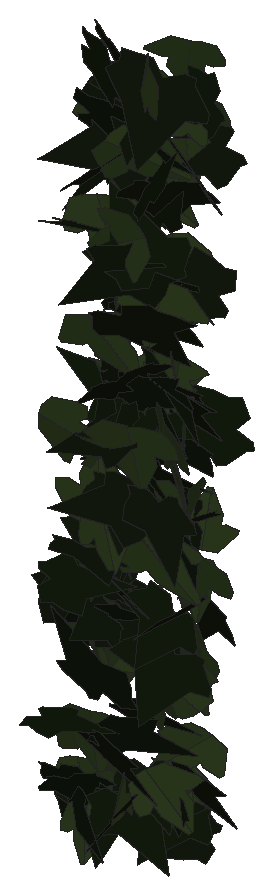
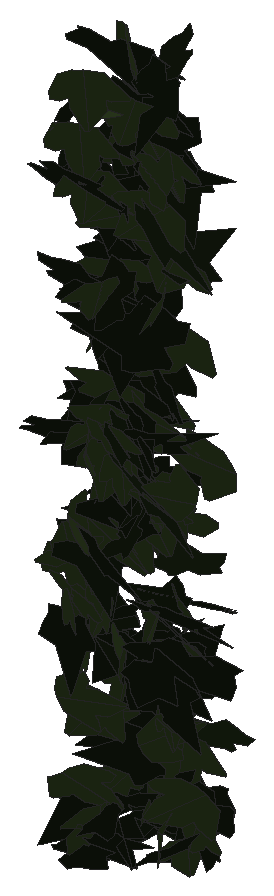
# SketchUp Ruby script. Lengths in inches.
U = 1.inch
M = Sketchup.active_model
def pt(a) = Geom::Point3d.new(a.map { |v| v * U })
def face(e, loops, mat)
  f = e.add_face(loops[0].map { |a| pt(a) })
  loops[1..].each { |l| e.add_face(l.map { |a| pt(a) }).erase! }
  f.material = f.back_material = mat if mat
  f
end
# faces: each face lists its corners as indices into pts; further lists are holes
def faces(e, pts, list, mat = nil) = list.each { |f| face(e, (f[0].is_a?(Array) ? f : [f]).map { |l| l.map { |i| pts[i] } }, mat) }
# xy, xz, yz: faces in a plane at the given z, y or x. An outline is a flat list of corners, or four numbers for a rectangle; further outlines are holes
def ring(l) = l.size == 4 ? [[l[0], l[1]], [l[2], l[1]], [l[2], l[3]], [l[0], l[3]]] : l.each_slice(2).to_a
def flat(e, list, mat, &to3) = list.each { |f| face(e, (f[0].is_a?(Array) ? f : [f]).map { |l| ring(l).map { |u, v| to3.(u, v) } }, mat) }
def xy(e, z, list, mat = nil) = flat(e, list, mat) { |x, y| [x, y, z] }
def xz(e, y, list, mat = nil) = flat(e, list, mat) { |x, z| [x, y, z] }
def yz(e, x, list, mat = nil) = flat(e, list, mat) { |y, z| [x, y, z] }
def lines(e, pts, list) = list.each { |a, b| e.add_line(pt(pts[a]), pt(pts[b])) }
# prism: a flat outline (further loops are holes) pulled along v
def prism(e, loops, v, mat = nil)
  f = face(e, loops, mat); d = Geom::Vector3d.new(v.map { |x| x * U })
  f.pushpull(f.normal.samedirection?(d) ? d.length : -d.length)
end
def box(e, o, s, mat = nil) = prism(e, [[o, [o[0] + s[0], o[1], o[2]], [o[0] + s[0], o[1] + s[1], o[2]], [o[0], o[1] + s[1], o[2]]]], [0, 0, s[2]], mat)
def at(x, y, z, deg = 0) = Geom::Transformation.translation(pt([x, y, z])) * Geom::Transformation.rotation(ORIGIN, Z_AXIS, deg.degrees)
def axes(o, x, y, z) = Geom::Transformation.new([*x, 0, *y, 0, *z, 0, *pt(o).to_a, 1])
def part(name) = M.definitions.add(name)
# library, detail: a bought-in or finely detailed component or shape, given as its bounding box
def library(name, o, s) = part(name).tap { |d| box(d.entities, o, s) }
def detail(e, o, s) = box(e.add_group.entities, o, s)
def put(e, d, t, mat = nil) = e.add_instance(d, t).tap { |i| i.material = mat if mat }
def group(e, t, mat = nil) = e.add_group.tap { |g| g.transformation = t; g.material = mat if mat }.entities
root = M.entities
M.materials.add("1026 AP 7946 SUNNY SIDE UP").color = [254, 231, 186]
M.materials.add("efeu1").color = [18, 25, 13]
M.materials.add("efeu2").color = [43, 57, 29]
c1 = part("ivyleaf_10")
p = [[0,0.5,-0.03],[-0.0625,2.02,-0.43],[-0.19,2.01,-0.46],[-0.54,1.05,-0.29],[-0.52,0.625,-0.18],[-0.83,0.76,-0.28],
  [-1.16,0.64,-0.33],[-1.15,0.33,-0.24],[-0.77,-0.39,0.02],[-0.3,-0.51,0.16],[0.04,-0.48,0.23],[-0.02,2.01,-0.4375],
  [-0.06,2.01,-0.43],[0.04,-0.49,0.23],[0.67,-0.49,0.14],[1.38,0.36,-0.2],[1.375,0.51,-0.24],[0.81,0.65,-0.19],
  [0.62,0.59,-0.15],[0.6,1.09,-0.28],[0.5,1.23,-0.31]]
faces(c1.entities,p,[[0,1,2,3,4,5,6,7,8,9,10],[11,12,0,13,14,15,16,17,18,19,20]],"efeu2")
c2 = part("ivyleaf_9")
p = [[1.54,2.16,1.25],[1.36,2.04,1.19],[-0.21,0.99,0.68],[-0.71,1.11,0.82],[-0.85,0.86,0.67],[-0.8,0.17,0.21],
  [-0.9,-0.01,0.1],[-0.67,-0.16,-0.02],[-0.08,-0.08,-0.05],[-0.03,-0.6,-0.4],[0.65,-0.88,-0.66],[0.83,-0.6,-0.49],
  [1.29,-0.42,-0.43],[1.8125,-0.07,-0.26],[1.21,0.44,0.15]]
faces(c2.entities,p,[[0,1,2,3,4,5,6,7,8,9,10,11,12,13,14]],"efeu1")
put(root,c1,axes([141.98,211.67,268.41],[0.3411,-0.04466,0.11048],[0.16001,-0.03763,-0.22788],[0.08887,0.23916,-0.01374]),"1026 AP 7946 SUNNY SIDE UP")
put(root,c2,axes([142.37,212.03,271.69],[-0.51179,-0.04689,0.03116],[-0.02985,-0.07688,-0.33075],[0.08274,-0.31774,0.07342]),"1026 AP 7946 SUNNY SIDE UP")
put(root,c2,axes([142.38,212.01,270.58],[0.16585,0.07044,-0.27143],[-0.35182,-0.13992,-0.13143],[-0.24626,0.24734,0.00497]),"1026 AP 7946 SUNNY SIDE UP")
put(root,c2,axes([142.32,212.13,270.93],[-0.05032,0.15512,-0.27609],[0.02205,-0.26931,-0.16335],[-0.4876,-0.02818,0.02111]),"1026 AP 7946 SUNNY SIDE UP")
put(root,c1,axes([141.97,211.8,268.92],[-0.39891,0.00207,-0.21595],[0.3263,-0.0443,-0.25942],[-0.04686,-0.3261,0.03193]),"1026 AP 7946 SUNNY SIDE UP")
put(root,c2,axes([142.06,211.26,268.57],[0.37583,0.06079,-0.02788],[-0.03131,-0.03229,-0.25282],[-0.10006,0.2384,-0.02562]),"1026 AP 7946 SUNNY SIDE UP")
put(root,c1,axes([142.29,211.69,270.94],[-0.40485,-0.03673,0.02647],[-0.03461,-0.02825,-0.26688],[0.06162,-0.25723,0.02398]),"1026 AP 7946 SUNNY SIDE UP")
put(root,c2,axes([142.41,211.94,271.52],[-0.39007,0.07794,-0.04071],[0.04506,-0.0412,-0.26629],[-0.13014,-0.24787,0.02982]),"1026 AP 7946 SUNNY SIDE UP")
put(root,c2,axes([142.42,212.125,277.55],[-0.42812,0.2333,-0.19837],[0.19927,-0.14921,-0.36919],[-0.43335,-0.29909,0.0262]),"1026 AP 7946 SUNNY SIDE UP")
put(root,c2,axes([141.96,211.89,271.05],[-0.1553,-0.19578,-0.34367],[0.27144,0.28452,-0.22376],[0.5426,-0.19837,0.01357]),"1026 AP 7946 SUNNY SIDE UP")
put(root,c1,axes([142.34,212.11,269.78],[0.03474,0.09893,0.29942],[-0.08598,-0.2849,0.10271],[0.47419,-0.0589,-0.00331]),"1026 AP 7946 SUNNY SIDE UP")
put(root,c1,axes([142.28,211.88,270.18],[-0.05171,-0.25295,-0.0237],[0.01452,0.02055,-0.26258],[0.39892,-0.03354,0.00649]),"1026 AP 7946 SUNNY SIDE UP")
put(root,c1,axes([142.18,211.77,273.24],[-0.02523,-0.13468,0.29495],[0.07676,0.28296,0.14122],[-0.49266,0.05099,0.0069]),"1026 AP 7946 SUNNY SIDE UP")
put(root,c1,axes([141.92,211.34,273.64],[-0.07651,0.00007,-0.36728],[0.49858,-0.1645,-0.04558],[-0.25629,-0.32002,0.02098]),"1026 AP 7946 SUNNY SIDE UP")
put(root,c2,axes([141.99,211.02,269.45],[0.23151,-0.20375,0.03077],[0.30705,0.12572,-0.1034],[0.10365,0.08268,0.23759]),"1026 AP 7946 SUNNY SIDE UP")
put(root,c2,axes([142.03,211.14,271.4375],[0.3609,-0.09301,-0.09777],[0.13489,0.24816,-0.03558],[0.1588,0.00058,0.25243]),"1026 AP 7946 SUNNY SIDE UP")
put(root,c2,axes([142.54,211.94,273.32],[-0.23259,0.23044,-0.01208],[-0.00128,-0.016,-0.28203],[-0.36292,-0.14763,0.00874]),"1026 AP 7946 SUNNY SIDE UP")
put(root,c2,axes([142.34,211.07,268.62],[0.23158,0.2003,-0.03003],[-0.01105,-0.03236,-0.25594],[-0.31833,0.14683,-0.01296]),"1026 AP 7946 SUNNY SIDE UP")
put(root,c1,axes([142.28,211.64,271.64],[0.29083,-0.15606,0.10948],[0.13347,-0.06553,-0.24965],[0.26606,0.20346,0.00557]),"1026 AP 7946 SUNNY SIDE UP")
put(root,c1,axes([142.48,211.77,270.63],[-0.40923,-0.15968,0.0214],[-0.00811,-0.03291,-0.31367],[0.25326,-0.25908,0.02454]),"1026 AP 7946 SUNNY SIDE UP")
put(root,c2,axes([142.11,211.33,268.22],[-0.00991,-0.02689,-0.31801],[0.48409,-0.03418,-0.00361],[-0.05307,-0.30671,0.02646]),"1026 AP 7946 SUNNY SIDE UP")
put(root,c1,axes([142.35,211.42,267.98],[0.20432,0.27023,-0.07488],[-0.02966,-0.07319,-0.30898],[-0.43965,0.13052,-0.01395]),"1026 AP 7946 SUNNY SIDE UP")
put(root,c2,axes([142.55,211.55,276.59],[-0.45066,-0.04883,0.00443],[0.07538,-0.28465,-0.03772],[0.01629,-0.03374,0.29714]),"1026 AP 7946 SUNNY SIDE UP")
put(root,c1,axes([142.36,211.65,270.33],[-0.09142,0.24804,-0.03639],[0.00938,-0.03632,-0.26266],[-0.39417,-0.05839,0.00219]),"1026 AP 7946 SUNNY SIDE UP")
put(root,c2,axes([142.32,211.8,268.09],[-0.12544,-0.31489,0.04124],[-0.00584,-0.0422,-0.33483],[0.49945,-0.07958,0.00644]),"1026 AP 7946 SUNNY SIDE UP")
put(root,c1,axes([142.46,211.41,269.37],[-0.52293,-0.04642,-0.00997],[0.02694,-0.05566,-0.34115],[0.06943,-0.32801,0.05729]),"1026 AP 7946 SUNNY SIDE UP")
put(root,c1,axes([142.5,211.71,268.19],[-0.02876,0.15992,-0.25655],[-0.04368,0.24839,0.16727],[0.46451,0.03326,-0.00015]),"1026 AP 7946 SUNNY SIDE UP")
put(root,c1,axes([142.35,211.9375,270.78],[0.35241,0.13023,-0.00815],[0.00541,-0.02308,-0.26624],[-0.20516,0.2231,-0.02102]),"1026 AP 7946 SUNNY SIDE UP")
put(root,c1,axes([142.14,212.2,278.06],[-0.10439,-0.02513,0.32624],[0.45519,-0.13836,0.05037],[0.20625,0.29264,0.05394]),"1026 AP 7946 SUNNY SIDE UP")
put(root,c2,axes([142.39,211.5,270.93],[0.30046,0.17784,-0.00707],[0.00972,-0.01818,-0.26842],[-0.27974,0.19038,-0.01693]),"1026 AP 7946 SUNNY SIDE UP")
put(root,c1,axes([142.51,211.76,273.21],[0.01338,-0.31658,0.13614],[0.00947,-0.13383,-0.32703],[0.54043,0.01018,0.00236]),"1026 AP 7946 SUNNY SIDE UP")
put(root,c2,axes([142.79,211.91,273.95],[-0.333,-0.21274,-0.0949],[-0.1267,-0.04771,0.3081],[-0.341,0.22547,-0.02179]),"1026 AP 7946 SUNNY SIDE UP")
put(root,c1,axes([142.45,212,271.54],[-0.2126,0.22431,-0.02991],[0.00855,-0.03207,-0.26973],[-0.35581,-0.1348,0.01138]),"1026 AP 7946 SUNNY SIDE UP")
put(root,c1,axes([142.28,211.74,276.72],[0.5058,0.00687,0.14965],[0.22859,-0.01239,-0.33121],[-0.00182,0.35271,-0.01248]),"1026 AP 7946 SUNNY SIDE UP")
put(root,c1,axes([142.34,212.05,277.56],[-0.43096,0.00456,-0.18907],[0.28373,-0.05432,-0.27927],[-0.05342,-0.32536,0.04202]),"1026 AP 7946 SUNNY SIDE UP")
put(root,c2,axes([142.35,211.76,274.55],[-0.04657,0.15349,0.28758],[0.09403,-0.2718,0.15941],[0.49079,0.06664,-0.00325]),"1026 AP 7946 SUNNY SIDE UP")
put(root,c2,axes([142.5,211.71,279.25],[0.42137,-0.10113,-0.20957],[-0.31287,0.0455,-0.29389],[0.17071,0.33301,-0.02133]),"1026 AP 7946 SUNNY SIDE UP")
put(root,c1,axes([142.48,211.83,276.11],[-0.05506,0.28152,-0.16174],[0.02936,-0.1575,-0.29318],[-0.50723,-0.03968,0.00059]),"1026 AP 7946 SUNNY SIDE UP")
put(root,c2,axes([142.77,211.8,277.84],[-0.0214,-0.15522,-0.31691],[-0.07455,-0.3032,0.15845],[-0.53539,0.04842,-0.0094]),"1026 AP 7946 SUNNY SIDE UP")
put(root,c1,axes([142.54,211.74,278.22],[0.52281,-0.1236,-0.00956],[-0.02872,-0.02459,-0.36432],[0.19269,0.33169,-0.02835]),"1026 AP 7946 SUNNY SIDE UP")
put(root,c2,axes([142.58,211.53,270.92],[-0.15347,-0.1387,0.20366],[-0.09559,-0.1931,-0.17095],[0.36854,-0.10784,0.04047]),"1026 AP 7946 SUNNY SIDE UP")
put(root,c2,axes([142.78,211.1875,277.79],[-0.02929,0.36162,0.00368],[-0.01242,0.00111,-0.37294],[-0.56849,-0.01866,0.00796]),"1026 AP 7946 SUNNY SIDE UP")
put(root,c1,axes([142.94,211.71,274.18],[0.15447,0.03666,0.32107],[-0.48995,0.04831,0.09568],[-0.05576,-0.32299,0.0488]),"1026 AP 7946 SUNNY SIDE UP")
put(root,c2,axes([142.83,212.26,273.84],[-0.39672,0.13381,-0.09281],[0.10282,-0.06959,-0.29306],[-0.2326,-0.25898,0.02876]),"1026 AP 7946 SUNNY SIDE UP")
put(root,c1,axes([142.77,211.67,272.76],[-0.31169,-0.15376,0.10483],[-0.07505,-0.10281,-0.25425],[0.28083,-0.19813,0.0484]),"1026 AP 7946 SUNNY SIDE UP")
put(root,c2,axes([142.87,211.0625,270.16],[0.24883,-0.14306,0.30101],[-0.30423,0.22095,0.22008],[-0.41268,-0.24914,0.01925]),"1026 AP 7946 SUNNY SIDE UP")
put(root,c2,axes([142.45,211.3,271.96],[-0.10405,-0.24607,0.08055],[0.29188,-0.10239,-0.16774],[0.28316,0.01512,0.20251]),"1026 AP 7946 SUNNY SIDE UP")
put(root,c1,axes([142.68,211.29,272.61],[0.58544,0.09555,0.0268],[-0.05453,0.03324,0.39396],[0.14562,-0.37171,0.03979]),"1026 AP 7946 SUNNY SIDE UP")
put(root,c2,axes([142.85,212.28,274.3],[-0.25362,0.16214,-0.16063],[0.15152,-0.12481,-0.23574],[-0.32072,-0.18719,0.01565]),"1026 AP 7946 SUNNY SIDE UP")
put(root,c1,axes([142.6,211.33,275.3],[-0.48086,-0.09389,-0.16806],[0.26727,-0.0064,-0.32556],[0.12544,-0.3463,0.04941]),"1026 AP 7946 SUNNY SIDE UP")
put(root,c2,axes([142.47,211.625,271.43],[0.1434,-0.16128,0.19188],[0.18335,-0.1478,-0.1906],[0.34251,0.14664,0.0217]),"1026 AP 7946 SUNNY SIDE UP")
put(root,c2,axes([143.125,211.2,273.98],[-0.44703,0.18032,0.0289],[-0.06504,-0.01503,-0.34506],[-0.27922,-0.28518,0.03412]),"1026 AP 7946 SUNNY SIDE UP")
put(root,c2,axes([142.62,212.15,272.87],[0.32789,-0.20444,-0.06832],[-0.09814,0.02914,-0.29979],[0.3228,0.21652,-0.02175]),"1026 AP 7946 SUNNY SIDE UP")
put(root,c1,axes([142.85,212.12,273.74],[-0.18542,-0.24817,-0.01169],[0.03632,0,-0.28224],[0.38884,-0.11834,0.02079]),"1026 AP 7946 SUNNY SIDE UP")
put(root,c2,axes([142.65,211.17,279.41],[0.42453,-0.20228,-0.20018],[-0.21595,0.13801,-0.34583],[0.38313,0.30193,0.02689]),"1026 AP 7946 SUNNY SIDE UP")
put(root,c2,axes([142.4375,211.87,275.48],[0.18233,0.0042,0.32775],[0.49802,0.03045,-0.11917],[-0.04724,0.33722,0.00866]),"1026 AP 7946 SUNNY SIDE UP")
put(root,c2,axes([142.55,211.94,269.41],[0.32148,-0.03205,0.15256],[0.23518,0.00104,-0.21223],[0.03984,0.25255,0.02173]),"1026 AP 7946 SUNNY SIDE UP")
put(root,c2,axes([142.39,211.53,278.24],[0.42811,-0.09631,0.2413],[0.32042,-0.12224,-0.29582],[0.2378,0.33809,-0.03582]),"1026 AP 7946 SUNNY SIDE UP")
put(root,c1,axes([142.78,211.22,272.62],[0.1726,0.34685,-0.00196],[0.01315,-0.0067,-0.37468],[-0.54526,0.10963,-0.00965]),"1026 AP 7946 SUNNY SIDE UP")
put(root,c1,axes([142.92,212.35,274.24],[0.40387,-0.08194,-0.06729],[-0.10099,0.01196,-0.27755],[0.12961,0.26464,-0.00659]),"1026 AP 7946 SUNNY SIDE UP")
put(root,c2,axes([142.63,211.21,269.27],[0.51085,-0.07542,-0.0265],[-0.04665,-0.0162,-0.34291],[0.11606,0.32546,-0.0212]),"1026 AP 7946 SUNNY SIDE UP")
put(root,c1,axes([142.85,212.21,270.93],[-0.07311,0.03614,-0.29137],[0.03943,-0.28514,-0.04342],[-0.44693,-0.03107,0.04384]),"1026 AP 7946 SUNNY SIDE UP")
put(root,c1,axes([142.88,211.55,268.53],[-0.02502,0.1318,-0.27965],[0.00756,-0.27243,-0.13778],[-0.47548,-0.01127,0.01253]),"1026 AP 7946 SUNNY SIDE UP")
put(root,c2,axes([142.61,211.96,272.98],[0.33222,-0.03267,0.17333],[0.26798,0.00907,-0.21837],[0.0312,0.27005,0.02991]),"1026 AP 7946 SUNNY SIDE UP")
put(root,c1,axes([143.35,212.03,272.53],[-0.17515,0.06561,0.29562],[-0.46163,-0.00862,-0.11557],[-0.02444,-0.30735,0.06446]),"1026 AP 7946 SUNNY SIDE UP")
put(root,c2,axes([143.21,211.79,274.45],[0.20487,0.23969,-0.21729],[-0.32968,-0.10934,-0.26039],[-0.38049,0.22379,0.10863]),"1026 AP 7946 SUNNY SIDE UP")
put(root,c2,axes([142.92,211.42,272.91],[-0.11946,-0.26106,0.005],[0.01547,-0.00946,-0.27987],[0.41031,-0.07565,0.01201]),"1026 AP 7946 SUNNY SIDE UP")
put(root,c2,axes([143.11,211.38,268.44],[-0.22553,0.17436,-0.20678],[0.15815,-0.17674,-0.2321],[-0.38827,-0.17327,0.02557]),"1026 AP 7946 SUNNY SIDE UP")
put(root,c2,axes([142.84,211.59,268.26],[-0.00992,-0.25502,-0.21134],[0.03536,0.20291,-0.26123],[0.51199,-0.01896,0.01394]),"1026 AP 7946 SUNNY SIDE UP")
put(root,c2,axes([142.77,211.92,273.1],[0.26626,-0.20696,0.05003],[0.04434,-0.04118,-0.27569],[0.33174,0.17162,-0.0033]),"1026 AP 7946 SUNNY SIDE UP")
put(root,c2,axes([143.11,211.12,274.76],[0.1498,0.36089,0.0399],[0.0277,0.03328,-0.38422],[-0.56971,0.09651,-0.00819]),"1026 AP 7946 SUNNY SIDE UP")
put(root,c2,axes([142.98,211.63,278.86],[-0.4127,-0.10195,-0.20118],[0.29913,0.0465,-0.28899],[0.17307,-0.32347,0.01974]),"1026 AP 7946 SUNNY SIDE UP")
put(root,c2,axes([142.6875,212.01,274.12],[0.04944,-0.0621,-0.34731],[0.53848,0.004,0.0322],[-0.00271,-0.33822,0.0621]),"1026 AP 7946 SUNNY SIDE UP")
put(root,c1,axes([143.32,211.11,276.93],[0.30526,-0.13942,-0.26253],[-0.3263,0.14654,-0.24537],[0.31804,0.28417,0.00023]),"1026 AP 7946 SUNNY SIDE UP")
put(root,c2,axes([143.29,211.57,273.91],[-0.30112,-0.05691,0.2021],[-0.23429,-0.14563,-0.1939],[0.22042,-0.23255,0.06999]),"1026 AP 7946 SUNNY SIDE UP")
put(root,c2,axes([143.44,212.2,272.39],[-0.15385,-0.01867,-0.30228],[-0.46213,0.00458,0.10073],[-0.00245,0.30916,-0.01793]),"1026 AP 7946 SUNNY SIDE UP")
put(root,c2,axes([142.89,211.82,270.91],[-0.1516,-0.22957,-0.2438],[0.19534,0.20165,-0.25388],[0.47865,-0.155,0.02639]),"1026 AP 7946 SUNNY SIDE UP")
put(root,c2,axes([143.32,211.25,272.96],[-0.07819,-0.15357,-0.27986],[-0.07776,-0.26684,0.1637],[-0.48327,0.06778,0.01894]),"1026 AP 7946 SUNNY SIDE UP")
put(root,c2,axes([143.14,211.71,275.52],[0.38505,0.11512,-0.17386],[-0.22912,-0.08767,-0.27886],[-0.22635,0.28457,-0.01348]),"1026 AP 7946 SUNNY SIDE UP")
put(root,c1,axes([143.13,211.97,273.74],[-0.30955,-0.25305,-0.06923],[0.08645,0.04042,-0.32952],[0.40192,-0.20358,0.01756]),"1026 AP 7946 SUNNY SIDE UP")
put(root,c1,axes([143.1,212.21,271.65],[-0.31791,0.23285,-0.04087],[0.0187,-0.04386,-0.3173],[-0.37129,-0.20158,0.01902]),"1026 AP 7946 SUNNY SIDE UP")
put(root,c2,axes([143,211.86,268.63],[-0.08778,-0.22216,-0.11736],[0.09219,0.10049,-0.23349],[0.38067,-0.07556,0.02948]),"1026 AP 7946 SUNNY SIDE UP")
put(root,c1,axes([142.93,211.77,278.77],[0.57786,0.08581,0.12172],[0.19352,-0.01227,-0.38686],[-0.12241,0.38568,-0.03702]),"1026 AP 7946 SUNNY SIDE UP")
put(root,c1,axes([143.51,212.33,270.13],[-0.13956,0.00031,-0.29635],[-0.43363,0.08558,0.08825],[0.12872,0.28863,-0.02401]),"1026 AP 7946 SUNNY SIDE UP")
put(root,c2,axes([143.4,211.16,276.56],[0.02318,0.05078,-0.34985],[-0.11634,-0.33176,-0.05631],[-0.5277,0.07537,-0.00295]),"1026 AP 7946 SUNNY SIDE UP")
put(root,c2,axes([143.43,211.85,268.46],[0.07624,-0.01118,-0.30355],[-0.46212,0.02161,-0.05055],[0.0364,0.29777,-0.00598]),"1026 AP 7946 SUNNY SIDE UP")
put(root,c2,axes([143.27,212.2,268.06],[-0.38352,-0.18896,0.00854],[0.01031,-0.02371,-0.31713],[0.29731,-0.24293,0.02201]),"1026 AP 7946 SUNNY SIDE UP")
put(root,c2,axes([142.9,211.24,269.43],[0.3447,0.11968,0.19136],[0.28681,0.048,-0.25427],[-0.19452,0.28285,-0.03582]),"1026 AP 7946 SUNNY SIDE UP")
put(root,c1,axes([142.85,211.88,277.32],[0.27736,0.10289,0.28016],[0.37975,0.12406,-0.20946],[-0.25306,0.29894,-0.00725]),"1026 AP 7946 SUNNY SIDE UP")
put(root,c2,axes([143.36,211.71,276.99],[0.11608,-0.0077,0.32516],[-0.12848,0.31268,0.02937],[-0.47961,-0.08563,0.07083]),"1026 AP 7946 SUNNY SIDE UP")
put(root,c1,axes([143.14,212.25,276.25],[0.16586,0.26853,-0.01226],[0.00665,-0.01608,-0.29714],[-0.42272,0.10511,-0.00949]),"1026 AP 7946 SUNNY SIDE UP")
put(root,c1,axes([143.49,212.0625,269.76],[0.24655,0.08916,0.24813],[-0.36597,-0.06858,0.18223],[0.16896,-0.27866,0.03264]),"1026 AP 7946 SUNNY SIDE UP")
put(root,c1,axes([143.34,212.31,279.22],[-0.39099,-0.17117,0.02507],[-0.01086,-0.03444,-0.31017],[0.27185,-0.24755,0.02366]),"1026 AP 7946 SUNNY SIDE UP")
put(root,c1,axes([143.2,212.18,268.5],[0.17883,0.28654,-0.05804],[-0.00937,-0.05991,-0.3175],[-0.45958,0.11272,-0.01611]),"1026 AP 7946 SUNNY SIDE UP")
put(root,c2,axes([142.93,212.11,276.11],[0.30848,-0.21146,0.15017],[0.12353,-0.1268,-0.29674],[0.38562,0.20978,-0.02507]),"1026 AP 7946 SUNNY SIDE UP")
put(root,c1,axes([143.16,212.24,270.11],[-0.4456,0.03985,-0.13568],[0.19639,-0.05327,-0.29326],[-0.09162,-0.30802,0.03128]),"1026 AP 7946 SUNNY SIDE UP")
put(root,c2,axes([143.43,212.01,272.35],[0.03677,0.32914,-0.04604],[-0.03454,-0.04504,-0.33966],[-0.52156,0.02619,0.01925]),"1026 AP 7946 SUNNY SIDE UP")
put(root,c1,axes([142.99,211.33,278.09],[-0.24648,-0.10842,-0.31739],[0.44421,0.12514,-0.1931],[0.25591,-0.32164,0.02948]),"1026 AP 7946 SUNNY SIDE UP")
put(root,c1,axes([143.39,212.36,278.45],[-0.45962,-0.03081,0.05528],[-0.08014,-0.02849,-0.30207],[0.05559,-0.29585,0.02156]),"1026 AP 7946 SUNNY SIDE UP")
put(root,c2,axes([143.47,211.83,273.72],[0.2204,0.12084,-0.25189],[-0.34108,-0.11851,-0.18861],[-0.26156,0.25636,0.0337]),"1026 AP 7946 SUNNY SIDE UP")
put(root,c1,axes([143.33,211.53,270.17],[-0.39041,0.19565,0.03709],[-0.06398,0.00461,-0.32488],[-0.30588,-0.25069,0.02062]),"1026 AP 7946 SUNNY SIDE UP")
put(root,c1,axes([143.44,212.38,268.98],[0.31727,0.08336,-0.21334],[-0.2882,-0.0986,-0.22493],[-0.20159,0.27216,-0.01419]),"1026 AP 7946 SUNNY SIDE UP")
put(root,c1,axes([143.11,212.07,274.27],[0.14837,0.22322,0.21385],[0.16033,0.18026,-0.24791],[-0.45025,0.13774,-0.01781]),"1026 AP 7946 SUNNY SIDE UP")
put(root,c2,axes([143.56,211.25,276.53],[-0.51082,-0.1347,0.04996],[0.05553,0.04309,0.36156],[-0.21858,0.32574,-0.0249]),"1026 AP 7946 SUNNY SIDE UP")
put(root,c1,axes([143.31,212.26,277.77],[-0.32284,-0.21225,-0.01315],[0.09178,-0.04084,-0.29571],[0.32139,-0.20155,0.07124]),"1026 AP 7946 SUNNY SIDE UP")
put(root,c2,axes([143.32,211.83,275.92],[0.34466,0.14413,-0.12139],[-0.13745,-0.08244,-0.27003],[-0.25938,0.23521,-0.0182]),"1026 AP 7946 SUNNY SIDE UP")
put(root,c1,axes([143.39,212.26,268.2],[0.11175,0.14792,-0.23087],[-0.16511,-0.19899,-0.17015],[-0.3898,0.1267,0.00589]),"1026 AP 7946 SUNNY SIDE UP")
put(root,c1,axes([143.36,211.07,274.04],[-0.55017,-0.11526,-0.02767],[0.05609,-0.0249,-0.37797],[0.1772,-0.34999,0.03373]),"1026 AP 7946 SUNNY SIDE UP")
put(root,c1,axes([143.52,211.22,279.32],[-0.3174,0.29468,0.07588],[-0.24161,-0.02478,-0.33955],[-0.41127,-0.21287,0.14092]),"1026 AP 7946 SUNNY SIDE UP")
put(root,c1,axes([143.34,211.93,273.36],[-0.25001,0.30107,-0.01236],[-0.00895,-0.0185,-0.35058],[-0.47381,-0.15852,0.01314]),"1026 AP 7946 SUNNY SIDE UP")
put(root,c2,axes([143.39,211.85,271.1],[-0.19942,-0.26009,0.13926],[-0.08039,-0.12704,-0.29871],[0.45494,-0.13646,0.00826]),"1026 AP 7946 SUNNY SIDE UP")
put(root,c2,axes([143.63,212.2,267.75],[-0.23113,-0.17767,-0.13884],[-0.06125,-0.13729,0.23116],[-0.34429,0.1437,0.05208]),"1026 AP 7946 SUNNY SIDE UP")
put(root,c1,axes([143.16,211.9,274.64],[0.38835,0.12826,0.15954],[0.24025,0.03799,-0.28456],[-0.20419,0.28864,-0.03139]),"1026 AP 7946 SUNNY SIDE UP")
put(root,c1,axes([143.43,211.86,272.26],[-0.16533,-0.30101,-0.0897],[0.05753,0.0776,-0.3279],[0.48859,-0.11099,0.00826]),"1026 AP 7946 SUNNY SIDE UP")
put(root,c2,axes([143.73,212.45,277.85],[-0.51168,0.01705,0.08398],[-0.13016,-0.0338,-0.33373],[-0.01295,-0.33374,0.03611]),"1026 AP 7946 SUNNY SIDE UP")
put(root,c2,axes([143.6,211.64,271.24],[-0.03789,0.34431,-0.01482],[-0.00768,-0.01672,-0.35561],[-0.54195,-0.02383,0.00608]),"1026 AP 7946 SUNNY SIDE UP")
put(root,c2,axes([143.16,211.45,274.48],[0.3099,0.10057,0.17666],[0.26576,0.04084,-0.22531],[-0.16309,0.25766,-0.03146]),"1026 AP 7946 SUNNY SIDE UP")
put(root,c2,axes([143.47,211.57,277.53],[0.28132,0.25021,-0.11084],[-0.08167,-0.09675,-0.31716],[-0.42131,0.18583,-0.01253]),"1026 AP 7946 SUNNY SIDE UP")
put(root,c1,axes([143.46,212.17,270.85],[-0.26478,0.20727,-0.0067],[-0.01235,-0.01626,-0.27469],[-0.3259,-0.16778,0.01585]),"1026 AP 7946 SUNNY SIDE UP")
put(root,c2,axes([143.22,211.96,274.57],[0.15755,-0.29388,0.10404],[0.05235,-0.09711,-0.32043],[0.48667,0.10558,0.00079]),"1026 AP 7946 SUNNY SIDE UP")
put(root,c2,axes([143.26,212.13,268.61],[0.49414,-0.01517,-0.02187],[-0.03442,-0.01558,-0.32376],[0.02213,0.31458,-0.01524]),"1026 AP 7946 SUNNY SIDE UP")
put(root,c2,axes([143.21,211.9,274.24],[0.48944,-0.01799,0.04275],[0.06228,-0.03233,-0.31993],[0.03463,0.31236,-0.0288]),"1026 AP 7946 SUNNY SIDE UP")
put(root,c2,axes([143.59,212.28,271.16],[0.3093,-0.01337,-0.22923],[-0.35039,-0.01102,-0.20239],[0.00092,0.29673,-0.01611]),"1026 AP 7946 SUNNY SIDE UP")
put(root,c1,axes([143.32,211.62,268.67],[0.2411,0.25752,0.1592],[0.15019,0.12095,-0.3075],[-0.44648,0.17975,-0.01747]),"1026 AP 7946 SUNNY SIDE UP")
put(root,c1,axes([143.33,212.21,273.75],[0.04722,-0.02654,0.32284],[0.29758,-0.25009,-0.04195],[0.39526,0.19146,-0.00699]),"1026 AP 7946 SUNNY SIDE UP")
put(root,c1,axes([143.47,212.29,272.72],[0.14737,-0.1918,0.2301],[0.1292,-0.20923,-0.22077],[0.44588,0.12402,-0.01208]),"1026 AP 7946 SUNNY SIDE UP")
put(root,c1,axes([143.48,211.74,275.45],[-0.09894,0.2866,-0.11948],[0.01597,-0.11803,-0.30261],[-0.48685,-0.06212,0.01436]),"1026 AP 7946 SUNNY SIDE UP")
put(root,c1,axes([143.59,212.24,271.5],[0.00232,-0.27136,-0.00238],[0.00562,0.00079,-0.27953],[0.42665,0.00146,0.00369]),"1026 AP 7946 SUNNY SIDE UP")
put(root,c2,axes([143.37,210.92,275.875],[0.4991,0.19244,0.0337],[0.07486,-0.0179,-0.38029],[-0.29737,0.31848,-0.03919]),"1026 AP 7946 SUNNY SIDE UP")
put(root,c2,axes([143.71,211.03,277.71],[0.02432,0.1785,0.33295],[0.02396,0.32188,-0.18258],[-0.57866,0.02083,0.00643]),"1026 AP 7946 SUNNY SIDE UP")
put(root,c1,axes([143.75,211.34,274.12],[-0.38377,0.21936,0.17314],[-0.22968,0.08599,-0.33614],[-0.36746,-0.28285,0.02928]),"1026 AP 7946 SUNNY SIDE UP")
put(root,c1,axes([143.38,211.49,272.21],[-0.4359,-0.08455,-0.20871],[0.3413,-0.06171,-0.28047],[0.04679,-0.33748,0.10141]),"1026 AP 7946 SUNNY SIDE UP")
put(root,c1,axes([143.61,211.79,278.51],[-0.45594,-0.00667,0.09527],[0.06645,-0.2798,0.11405],[0.12983,0.1198,0.2762]),"1026 AP 7946 SUNNY SIDE UP")
put(root,c1,axes([143.56,211.43,276.05],[0.45838,0.15981,-0.05212],[-0.05421,-0.04402,-0.34201],[-0.25838,0.29274,-0.02071]),"1026 AP 7946 SUNNY SIDE UP")
put(root,c2,axes([143.64,211.58,270.66],[-0.34683,-0.25532,0.01066],[0.02979,-0.03187,-0.34589],[0.40079,-0.21857,0.03494]),"1026 AP 7946 SUNNY SIDE UP")
put(root,c1,axes([143.8,211.89,271.93],[-0.50602,0.00071,0.11049],[-0.16772,-0.0373,-0.32971],[0.01749,-0.33715,0.03472]),"1026 AP 7946 SUNNY SIDE UP")
put(root,c2,axes([144.05,211.91,276.02],[-0.32417,0.09771,0.22325],[-0.33758,0.04493,-0.23161],[-0.15862,-0.29531,0.03667]),"1026 AP 7946 SUNNY SIDE UP")
put(root,c1,axes([143.61,212.21,272.16],[0.24499,0.23891,-0.10866],[0.07369,0.09686,0.29411],[0.40486,-0.1622,0.01222]),"1026 AP 7946 SUNNY SIDE UP")
put(root,c2,axes([143.64,211.34,279.27],[-0.50483,-0.17152,-0.16171],[0.24176,0.04193,-0.37324],[0.27287,-0.35448,0.03151]),"1026 AP 7946 SUNNY SIDE UP")
put(root,c2,axes([143.7,212.02,277.54],[0.25663,-0.29983,0.09221],[-0.03729,0.09073,0.3515],[-0.49138,-0.16348,0.02148]),"1026 AP 7946 SUNNY SIDE UP")
put(root,c2,axes([143.72,212.28,278.57],[-0.10919,-0.10277,0.28019],[-0.2018,-0.24074,-0.12861],[0.41118,-0.14544,0.01129]),"1026 AP 7946 SUNNY SIDE UP")
put(root,c1,axes([143.52,212.26,271.61],[0.41284,-0.09772,0.1194],[0.15133,-0.07306,-0.28711],[0.18503,0.27777,-0.03158]),"1026 AP 7946 SUNNY SIDE UP")
put(root,c2,axes([143.48,211.9,272.33],[0.08097,-0.24313,0.20935],[0.05738,-0.20137,-0.25716],[0.49634,0.06294,-0.00443]),"1026 AP 7946 SUNNY SIDE UP")
put(root,c2,axes([144.07,212.25,273.89],[-0.41607,0.00032,0.20496],[-0.29697,-0.10448,-0.25922],[0.09835,-0.31414,0.08438]),"1026 AP 7946 SUNNY SIDE UP")
put(root,c2,axes([143.5625,211.39,272.95],[0.00352,-0.32859,-0.0057],[-0.00052,0.00367,-0.3385],[0.51671,0.00224,-0.0003]),"1026 AP 7946 SUNNY SIDE UP")
